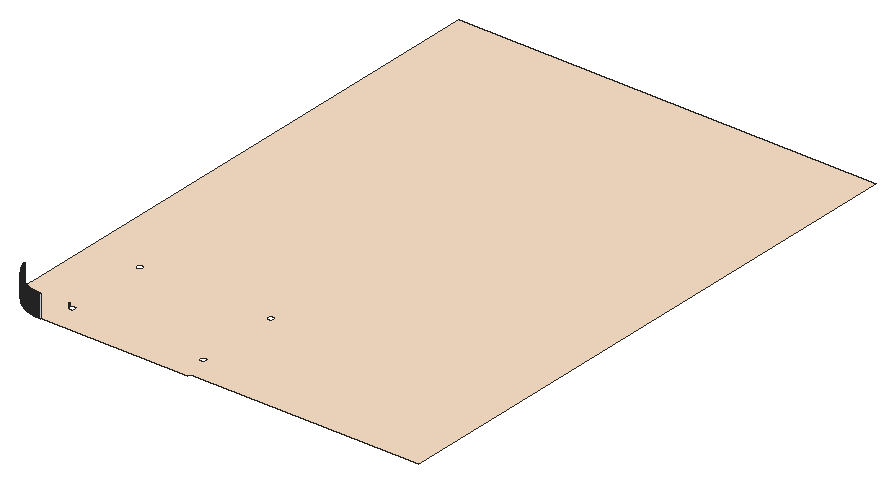
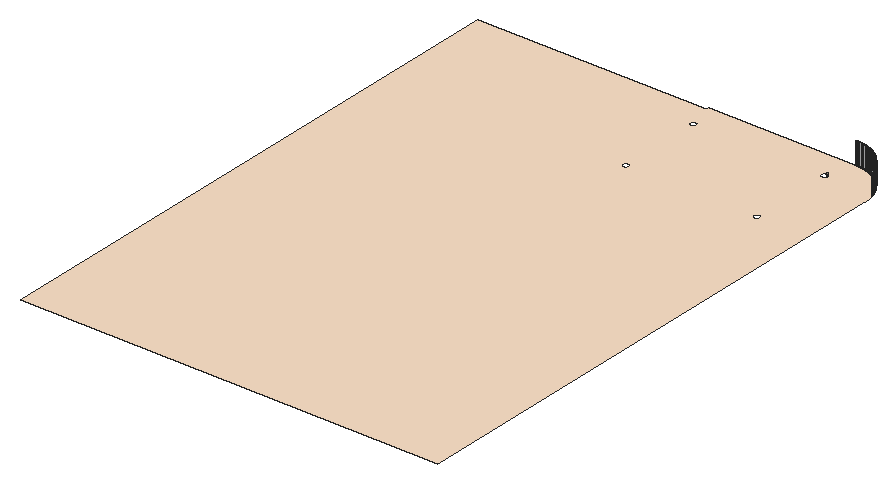
# SketchUp Ruby script. Lengths in inches.
U = 1.inch
M = Sketchup.active_model
def pt(a) = Geom::Point3d.new(a.map { |v| v * U })
def face(e, loops, mat)
  f = e.add_face(loops[0].map { |a| pt(a) })
  loops[1..].each { |l| e.add_face(l.map { |a| pt(a) }).erase! }
  f.material = f.back_material = mat if mat
  f
end
# faces: each face lists its corners as indices into pts; further lists are holes
def faces(e, pts, list, mat = nil) = list.each { |f| face(e, (f[0].is_a?(Array) ? f : [f]).map { |l| l.map { |i| pts[i] } }, mat) }
# xy, xz, yz: faces in a plane at the given z, y or x. An outline is a flat list of corners, or four numbers for a rectangle; further outlines are holes
def ring(l) = l.size == 4 ? [[l[0], l[1]], [l[2], l[1]], [l[2], l[3]], [l[0], l[3]]] : l.each_slice(2).to_a
def flat(e, list, mat, &to3) = list.each { |f| face(e, (f[0].is_a?(Array) ? f : [f]).map { |l| ring(l).map { |u, v| to3.(u, v) } }, mat) }
def xy(e, z, list, mat = nil) = flat(e, list, mat) { |x, y| [x, y, z] }
def xz(e, y, list, mat = nil) = flat(e, list, mat) { |x, z| [x, y, z] }
def yz(e, x, list, mat = nil) = flat(e, list, mat) { |y, z| [x, y, z] }
def lines(e, pts, list) = list.each { |a, b| e.add_line(pt(pts[a]), pt(pts[b])) }
# prism: a flat outline (further loops are holes) pulled along v
def prism(e, loops, v, mat = nil)
  f = face(e, loops, mat); d = Geom::Vector3d.new(v.map { |x| x * U })
  f.pushpull(f.normal.samedirection?(d) ? d.length : -d.length)
end
def box(e, o, s, mat = nil) = prism(e, [[o, [o[0] + s[0], o[1], o[2]], [o[0] + s[0], o[1] + s[1], o[2]], [o[0], o[1] + s[1], o[2]]]], [0, 0, s[2]], mat)
def at(x, y, z, deg = 0) = Geom::Transformation.translation(pt([x, y, z])) * Geom::Transformation.rotation(ORIGIN, Z_AXIS, deg.degrees)
def axes(o, x, y, z) = Geom::Transformation.new([*x, 0, *y, 0, *z, 0, *pt(o).to_a, 1])
def part(name) = M.definitions.add(name)
# library, detail: a bought-in or finely detailed component or shape, given as its bounding box
def library(name, o, s) = part(name).tap { |d| box(d.entities, o, s) }
def detail(e, o, s) = box(e.add_group.entities, o, s)
def put(e, d, t, mat = nil) = e.add_instance(d, t).tap { |i| i.material = mat if mat }
def group(e, t, mat = nil) = e.add_group.tap { |g| g.transformation = t; g.material = mat if mat }.entities
root = M.entities
M.materials.add("1122 AP 7994 PEACH ROSE").color = [254, 227, 201]
M.materials.add("[Quartz Light Grey]").color = [251, 251, 252]
xy(root,278.82,[[[44.6875,153,44.37,153.01,44.06,153.01,43.74,153.02,43.43,153.03,43.12,153.05,42.8,153.07,42.18,153.11,41.86,153.14,41.24,153.2,40.92,153.23,39.99,153.35,39.68,153.4,39.37,153.44,39.06,153.49,38.75,153.55,38.44,153.6,37.82,153.72,37.52,153.79,37.21,153.85,36.9,153.92,36.6,153.99,36.29,154.07,35.99,154.15,35.68,154.23,35.08,154.39,34.78,154.48,34.47,154.57,34.17,154.67,33.875,154.76,33.58,154.86,32.98,155.06,32.6875,155.17,32.39,155.28,31.81,155.5,31.51,155.62,30.93,155.86,30.65,155.99,30.36,156.11,30.07,156.24,29.79,156.37,29.5,156.51,29.22,156.64,28.9375,156.78,28.66,156.92,28.38,157.07,28.1,157.21,27.82,157.36,27.55,157.51,27.27,157.67,27,157.82,26.19,158.3,25.92,158.47,25.66,158.64,25.39,158.81,24.87,159.15,24.09,159.69,23.84,159.875,23.59,160.0625,23.33,160.25,23.08,160.4375,22.84,160.63,22.59,160.83,22.34,161.02,21.86,161.42,21.38,161.83,21.15,162.04,20.91,162.25,20.45,162.67,20.22,162.89,19.99,163.1,19.77,163.32,19.54,163.54,19.32,163.77,19.1,163.99,18.89,164.22,18.67,164.45,18.25,164.91,18.04,165.15,17.83,165.38,17.42,165.86,17.02,166.34,16.83,166.59,16.63,166.84,16.4375,167.08,16.25,167.33,16.0625,167.59,15.875,167.84,15.69,168.09,15.15,168.87,14.81,169.39,14.64,169.66,14.47,169.92,14.3,170.19,13.82,171,13.67,171.27,13.51,171.55,13.36,171.82,13.21,172.1,13.07,172.38,12.92,172.66,12.78,172.9375,12.64,173.22,12.51,173.5,12.37,173.79,12.24,174.07,12.11,174.36,11.99,174.65,11.86,174.93,11.62,175.51,11.5,175.81,11.28,176.39,11.17,176.6875,11.06,176.98,10.86,177.58,10.76,177.875,10.67,178.17,10.57,178.47,10.48,178.78,10.39,179.08,10.23,179.68,10.15,179.99,10.07,180.29,9.99,180.6,9.92,180.9,9.85,181.21,9.79,181.52,9.72,181.82,9.6,182.44,9.55,182.75,9.49,183.06,9.44,183.37,9.4,183.68,9.35,183.99,9.23,184.92,9.2,185.24,9.14,185.86,9.11,186.18,9.07,186.8,9.05,187.12,9.03,187.43,9.02,187.74,9.01,188.06,9.01,188.37,9,188.6875,9,645,366,645,366,156,171.19,156,171.19,153],[52.82,174,53.14,174,53.22,174.01,53.29,174.02,53.53,174.05,53.6,174.07,53.68,174.08,53.76,174.1,53.83,174.125,53.91,174.15,53.98,174.17,54.06,174.2,54.27,174.29,54.34,174.33,54.41,174.36,54.55,174.44,54.61,174.48,54.68,174.53,54.74,174.57,54.81,174.62,55.05,174.82,55.1,174.88,55.16,174.93,55.26,175.05,55.3125,175.11,55.36,175.17,55.41,175.24,55.45,175.3,55.5,175.37,55.54,175.43,55.62,175.57,55.65,175.64,55.6875,175.71,55.72,175.78,55.78,175.92,55.81,176,55.83,176.07,55.86,176.15,55.88,176.22,55.9,176.3,55.92,176.375,55.93,176.45,55.94,176.53,55.96,176.61,55.96,176.6875,55.97,176.76,55.98,176.84,55.98,177.16,55.97,177.24,55.96,177.3125,55.96,177.39,55.94,177.47,55.93,177.55,55.92,177.625,55.9,177.7,55.88,177.78,55.86,177.85,55.83,177.93,55.81,178,55.78,178.08,55.72,178.22,55.6875,178.29,55.65,178.36,55.62,178.43,55.54,178.57,55.5,178.63,55.45,178.7,55.41,178.76,55.36,178.83,55.3125,178.89,55.26,178.95,55.16,179.07,55.1,179.12,55.05,179.18,54.81,179.38,54.74,179.43,54.68,179.47,54.61,179.52,54.55,179.56,54.41,179.64,54.34,179.67,54.27,179.71,54.06,179.8,53.98,179.83,53.91,179.85,53.83,179.875,53.76,179.9,53.68,179.92,53.6,179.93,53.53,179.95,53.29,179.98,53.22,179.99,53.14,180,52.82,180,52.75,179.99,52.43,179.95,52.36,179.93,52.28,179.92,52.2,179.9,52.13,179.875,52.05,179.85,51.98,179.83,51.91,179.8,51.83,179.77,51.76,179.74,51.6875,179.71,51.62,179.67,51.55,179.64,51.41,179.56,51.35,179.52,51.28,179.47,51.22,179.43,51.15,179.38,50.97,179.23,50.86,179.12,50.8,179.07,50.6,178.83,50.55,178.76,50.51,178.7,50.46,178.63,50.42,178.57,50.34,178.43,50.31,178.36,50.27,178.29,50.18,178.08,50.15,178,50.13,177.93,50.1,177.85,50.08,177.78,50.0625,177.7,50.05,177.625,50.03,177.55,50.01,177.39,50,177.3125,49.99,177.24,49.99,177.16,49.98,177.08,49.98,176.92,49.99,176.84,49.99,176.76,50,176.6875,50.01,176.61,50.03,176.45,50.05,176.375,50.0625,176.3,50.08,176.22,50.1,176.15,50.13,176.07,50.15,176,50.18,175.92,50.27,175.71,50.31,175.64,50.34,175.57,50.42,175.43,50.46,175.37,50.51,175.3,50.55,175.24,50.6,175.17,50.8,174.93,50.86,174.88,50.97,174.77,51.15,174.62,51.22,174.57,51.28,174.53,51.35,174.48,51.41,174.44,51.55,174.36,51.62,174.33,51.6875,174.29,51.76,174.26,51.83,174.23,51.91,174.2,51.98,174.17,52.05,174.15,52.13,174.125,52.2,174.1,52.28,174.08,52.36,174.07,52.43,174.05,52.75,174.01],[164.84,246,165.16,246,165.24,246.01,165.3125,246.02,165.39,246.03,165.55,246.05,165.625,246.07,165.7,246.08,165.78,246.1,165.85,246.125,165.93,246.15,166,246.17,166.08,246.2,166.29,246.29,166.36,246.33,166.43,246.36,166.57,246.44,166.63,246.48,166.7,246.53,166.76,246.57,166.83,246.62,167.07,246.82,167.12,246.88,167.18,246.93,167.38,247.17,167.43,247.24,167.47,247.3,167.52,247.37,167.56,247.43,167.64,247.57,167.67,247.64,167.71,247.71,167.8,247.92,167.83,248,167.85,248.07,167.875,248.15,167.9,248.22,167.92,248.3,167.93,248.375,167.95,248.45,167.97,248.61,167.98,248.6875,167.99,248.76,168,248.84,168,249.16,167.99,249.24,167.98,249.3125,167.97,249.39,167.95,249.55,167.93,249.625,167.92,249.7,167.9,249.78,167.875,249.85,167.85,249.93,167.83,250,167.8,250.08,167.71,250.29,167.67,250.36,167.64,250.43,167.56,250.57,167.52,250.63,167.47,250.7,167.43,250.76,167.38,250.83,167.18,251.07,167.12,251.12,167.07,251.18,166.83,251.38,166.76,251.43,166.7,251.47,166.63,251.52,166.57,251.56,166.43,251.64,166.36,251.67,166.29,251.71,166.08,251.8,166,251.83,165.93,251.85,165.85,251.875,165.78,251.9,165.7,251.92,165.625,251.93,165.55,251.95,165.39,251.97,165.3125,251.98,165.24,251.99,165.16,252,164.84,252,164.76,251.99,164.6875,251.98,164.61,251.97,164.45,251.95,164.375,251.93,164.3,251.92,164.22,251.9,164.15,251.875,164.07,251.85,164,251.83,163.92,251.8,163.71,251.71,163.64,251.67,163.57,251.64,163.43,251.56,163.37,251.52,163.3,251.47,163.24,251.43,163.17,251.38,162.93,251.18,162.88,251.12,162.82,251.07,162.62,250.83,162.57,250.76,162.53,250.7,162.48,250.63,162.44,250.57,162.36,250.43,162.33,250.36,162.29,250.29,162.2,250.08,162.17,250,162.15,249.93,162.125,249.85,162.1,249.78,162.08,249.7,162.07,249.625,162.05,249.55,162.03,249.39,162.02,249.3125,162.01,249.24,162,249.16,162,248.84,162.01,248.76,162.02,248.6875,162.03,248.61,162.05,248.45,162.07,248.375,162.08,248.3,162.1,248.22,162.125,248.15,162.15,248.07,162.17,248,162.2,247.92,162.29,247.71,162.33,247.64,162.36,247.57,162.44,247.43,162.48,247.37,162.53,247.3,162.57,247.24,162.62,247.17,162.82,246.93,162.88,246.88,162.93,246.82,163.17,246.62,163.24,246.57,163.3,246.53,163.37,246.48,163.43,246.44,163.57,246.36,163.64,246.33,163.71,246.29,163.92,246.2,164,246.17,164.07,246.15,164.15,246.125,164.22,246.1,164.3,246.08,164.375,246.07,164.45,246.05,164.61,246.03,164.6875,246.02,164.76,246.01],[164.84,174,165.16,174,165.24,174.01,165.3125,174.02,165.39,174.03,165.55,174.05,165.625,174.07,165.7,174.08,165.78,174.1,165.85,174.125,165.93,174.15,166,174.17,166.08,174.2,166.29,174.29,166.36,174.33,166.43,174.36,166.57,174.44,166.63,174.48,166.7,174.53,166.76,174.57,166.83,174.62,167.07,174.82,167.12,174.88,167.18,174.93,167.38,175.17,167.43,175.24,167.47,175.3,167.52,175.37,167.56,175.43,167.64,175.57,167.67,175.64,167.71,175.71,167.8,175.92,167.83,176,167.85,176.07,167.875,176.15,167.9,176.22,167.92,176.3,167.93,176.375,167.95,176.45,167.97,176.61,167.98,176.6875,167.99,176.76,168,176.84,168,177.16,167.99,177.24,167.98,177.3125,167.97,177.39,167.95,177.55,167.93,177.625,167.92,177.7,167.9,177.78,167.875,177.85,167.85,177.93,167.83,178,167.8,178.08,167.71,178.29,167.67,178.36,167.64,178.43,167.56,178.57,167.52,178.63,167.47,178.7,167.43,178.76,167.38,178.83,167.18,179.07,167.12,179.12,167.07,179.18,166.83,179.38,166.76,179.43,166.7,179.47,166.63,179.52,166.57,179.56,166.43,179.64,166.36,179.67,166.29,179.71,166.08,179.8,166,179.83,165.93,179.85,165.85,179.875,165.78,179.9,165.7,179.92,165.625,179.93,165.55,179.95,165.39,179.97,165.3125,179.98,165.24,179.99,165.16,180,164.84,180,164.76,179.99,164.6875,179.98,164.61,179.97,164.45,179.95,164.375,179.93,164.3,179.92,164.22,179.9,164.15,179.875,164.07,179.85,164,179.83,163.92,179.8,163.71,179.71,163.64,179.67,163.57,179.64,163.43,179.56,163.37,179.52,163.3,179.47,163.24,179.43,163.17,179.38,162.93,179.18,162.88,179.12,162.82,179.07,162.62,178.83,162.57,178.76,162.53,178.7,162.48,178.63,162.44,178.57,162.36,178.43,162.33,178.36,162.29,178.29,162.2,178.08,162.17,178,162.15,177.93,162.125,177.85,162.1,177.78,162.08,177.7,162.07,177.625,162.05,177.55,162.03,177.39,162.02,177.3125,162.01,177.24,162,177.16,162,176.84,162.01,176.76,162.02,176.6875,162.03,176.61,162.05,176.45,162.07,176.375,162.08,176.3,162.1,176.22,162.125,176.15,162.15,176.07,162.17,176,162.2,175.92,162.29,175.71,162.33,175.64,162.36,175.57,162.44,175.43,162.48,175.37,162.53,175.3,162.57,175.24,162.62,175.17,162.82,174.93,162.88,174.88,162.93,174.82,163.17,174.62,163.24,174.57,163.3,174.53,163.37,174.48,163.43,174.44,163.57,174.36,163.64,174.33,163.71,174.29,163.92,174.2,164,174.17,164.07,174.15,164.15,174.125,164.22,174.1,164.3,174.08,164.375,174.07,164.45,174.05,164.61,174.03,164.6875,174.02,164.76,174.01],[52.82,246,53.14,246,53.22,246.01,53.29,246.02,53.53,246.05,53.6,246.07,53.68,246.08,53.76,246.1,53.83,246.125,53.91,246.15,53.98,246.17,54.06,246.2,54.27,246.29,54.34,246.33,54.41,246.36,54.55,246.44,54.61,246.48,54.68,246.53,54.74,246.57,54.81,246.62,55.05,246.82,55.1,246.88,55.16,246.93,55.26,247.05,55.3125,247.11,55.36,247.17,55.41,247.24,55.45,247.3,55.5,247.37,55.54,247.43,55.62,247.57,55.65,247.64,55.6875,247.71,55.72,247.78,55.78,247.92,55.81,248,55.83,248.07,55.86,248.15,55.88,248.22,55.9,248.3,55.92,248.375,55.93,248.45,55.94,248.53,55.96,248.61,55.96,248.6875,55.97,248.76,55.98,248.84,55.98,249.16,55.97,249.24,55.96,249.3125,55.96,249.39,55.94,249.47,55.93,249.55,55.92,249.625,55.9,249.7,55.88,249.78,55.86,249.85,55.83,249.93,55.81,250,55.78,250.08,55.72,250.22,55.6875,250.29,55.65,250.36,55.62,250.43,55.54,250.57,55.5,250.63,55.45,250.7,55.41,250.76,55.36,250.83,55.3125,250.89,55.26,250.95,55.16,251.07,55.1,251.12,55.05,251.18,54.81,251.38,54.74,251.43,54.68,251.47,54.61,251.52,54.55,251.56,54.41,251.64,54.34,251.67,54.27,251.71,54.06,251.8,53.98,251.83,53.91,251.85,53.83,251.875,53.76,251.9,53.68,251.92,53.6,251.93,53.53,251.95,53.29,251.98,53.22,251.99,53.14,252,52.82,252,52.75,251.99,52.43,251.95,52.36,251.93,52.28,251.92,52.2,251.9,52.13,251.875,52.05,251.85,51.98,251.83,51.91,251.8,51.83,251.77,51.76,251.74,51.6875,251.71,51.62,251.67,51.55,251.64,51.41,251.56,51.35,251.52,51.28,251.47,51.22,251.43,51.15,251.38,50.97,251.23,50.86,251.12,50.8,251.07,50.6,250.83,50.55,250.76,50.51,250.7,50.46,250.63,50.42,250.57,50.34,250.43,50.31,250.36,50.27,250.29,50.18,250.08,50.15,250,50.13,249.93,50.1,249.85,50.08,249.78,50.0625,249.7,50.05,249.625,50.03,249.55,50.01,249.39,50,249.3125,49.99,249.24,49.99,249.16,49.98,249.08,49.98,248.92,49.99,248.84,49.99,248.76,50,248.6875,50.01,248.61,50.03,248.45,50.05,248.375,50.0625,248.3,50.08,248.22,50.1,248.15,50.13,248.07,50.15,248,50.18,247.92,50.27,247.71,50.31,247.64,50.34,247.57,50.42,247.43,50.46,247.37,50.51,247.3,50.55,247.24,50.6,247.17,50.8,246.93,50.86,246.88,50.97,246.77,51.15,246.62,51.22,246.57,51.28,246.53,51.35,246.48,51.41,246.44,51.55,246.36,51.62,246.33,51.6875,246.29,51.76,246.26,51.83,246.23,51.91,246.2,51.98,246.17,52.05,246.15,52.13,246.125,52.2,246.1,52.28,246.08,52.36,246.07,52.43,246.05,52.75,246.01]]],"1122 AP 7994 PEACH ROSE")
xz(root,153,[[44.6875,278.82,45,297.82]],"[Quartz Light Grey]")
xz(root,153.01,[[44.06,278.82,44.37,297.82]],"[Quartz Light Grey]")
yz(root,49.98,[[176.92,278.82,177,281.82],[177,278.82,177.08,281.82]],"1122 AP 7994 PEACH ROSE")
yz(root,49.99,[[176.76,278.82,176.84,281.82],[177.16,278.82,177.24,281.82]],"1122 AP 7994 PEACH ROSE")
p = [[42.8,153.07,278.82],[43.12,153.05,278.82],[43.12,153.05,297.82],[42.8,153.07,297.82],[43.43,153.03,278.82],[43.43,153.03,297.82],
  [43.74,153.02,278.82],[43.74,153.02,297.82],[44.06,153.01,278.82],[44.06,153.01,297.82],[44.37,153.01,278.82],[44.6875,153,278.82],
  [44.6875,153,297.82],[44.37,153.01,297.82],[41.55,153.17,278.82],[41.86,153.14,278.82],[41.86,153.14,297.82],[41.55,153.17,297.82],
  [42.18,153.11,278.82],[42.18,153.11,297.82],[42.49,153.09,278.82],[42.49,153.09,297.82],[40.61,153.27,278.82],[40.92,153.23,278.82],
  [40.92,153.23,297.82],[40.61,153.27,297.82],[41.24,153.2,278.82],[41.24,153.2,297.82],[39.99,153.35,278.82],[40.3,153.31,278.82],
  [40.3,153.31,297.82],[39.99,153.35,297.82],[39.06,153.49,278.82],[39.37,153.44,278.82],[39.37,153.44,297.82],[39.06,153.49,297.82],
  [39.68,153.4,278.82],[39.68,153.4,297.82],[38.44,153.6,278.82],[38.75,153.55,278.82],[38.75,153.55,297.82],[38.44,153.6,297.82],
  [38.13,153.66,278.82],[38.13,153.66,297.82],[37.52,153.79,278.82],[37.82,153.72,278.82],[37.82,153.72,297.82],[37.52,153.79,297.82],
  [37.21,153.85,278.82],[37.21,153.85,297.82],[36.6,153.99,278.82],[36.9,153.92,278.82],[36.9,153.92,297.82],[36.6,153.99,297.82],
  [36.29,154.07,278.82],[36.29,154.07,297.82],[35.68,154.23,278.82],[35.99,154.15,278.82],[35.99,154.15,297.82],[35.68,154.23,297.82],
  [35.38,154.31,278.82],[35.38,154.31,297.82],[35.08,154.39,278.82],[35.08,154.39,297.82],[34.78,154.48,278.82],[34.78,154.48,297.82],
  [34.47,154.57,278.82],[34.47,154.57,297.82],[34.17,154.67,278.82],[34.17,154.67,297.82],[33.875,154.76,278.82],[33.875,154.76,297.82],
  [33.58,154.86,278.82],[33.58,154.86,297.82],[33.28,154.96,278.82],[33.28,154.96,297.82],[32.98,155.06,278.82],[32.98,155.06,297.82],
  [32.6875,155.17,278.82],[32.6875,155.17,297.82],[32.39,155.28,278.82],[32.39,155.28,297.82],[32.1,155.39,278.82],[32.1,155.39,297.82],
  [31.81,155.5,278.82],[31.81,155.5,297.82],[31.51,155.62,278.82],[31.51,155.62,297.82],[31.22,155.74,278.82],[31.22,155.74,297.82],
  [30.93,155.86,278.82],[30.93,155.86,297.82],[30.65,155.99,278.82],[30.65,155.99,297.82],[30.36,156.11,278.82],[30.36,156.11,297.82],
  [30.07,156.24,278.82],[30.07,156.24,297.82],[29.79,156.37,278.82],[29.79,156.37,297.82],[29.5,156.51,278.82],[29.5,156.51,297.82],
  [29.22,156.64,278.82],[29.22,156.64,297.82],[28.9375,156.78,278.82],[28.9375,156.78,297.82],[28.66,156.92,278.82],[28.66,156.92,297.82],
  [28.38,157.07,278.82],[28.38,157.07,297.82],[28.1,157.21,278.82],[28.1,157.21,297.82],[27.82,157.36,278.82],[27.82,157.36,297.82],
  [27.55,157.51,278.82],[27.55,157.51,297.82],[27.27,157.67,278.82],[27.27,157.67,297.82],[27,157.82,278.82],[27,157.82,297.82],
  [26.73,157.98,278.82],[26.73,157.98,297.82],[26.46,158.14,278.82],[26.46,158.14,297.82],[26.19,158.3,278.82],[26.19,158.3,297.82],
  [25.92,158.47,278.82],[25.92,158.47,297.82],[25.66,158.64,278.82],[25.66,158.64,297.82],[25.39,158.81,278.82],[25.39,158.81,297.82],
  [25.13,158.98,278.82],[25.13,158.98,297.82],[24.87,159.15,278.82],[24.87,159.15,297.82],[24.61,159.33,278.82],[24.61,159.33,297.82],
  [24.35,159.51,278.82],[24.35,159.51,297.82],[24.09,159.69,278.82],[24.09,159.69,297.82],[23.84,159.875,278.82],[23.84,159.875,297.82],
  [23.59,160.0625,278.82],[23.59,160.0625,297.82],[23.33,160.25,278.82],[23.33,160.25,297.82],[23.08,160.4375,278.82],[23.08,160.4375,297.82],
  [22.84,160.63,278.82],[22.84,160.63,297.82],[22.59,160.83,278.82],[22.59,160.83,297.82],[22.34,161.02,278.82],[22.34,161.02,297.82],
  [22.1,161.22,278.82],[22.1,161.22,297.82],[21.86,161.42,278.82],[21.86,161.42,297.82],[21.62,161.625,278.82],[21.62,161.625,297.82],
  [21.38,161.83,278.82],[21.38,161.83,297.82],[21.15,162.04,278.82],[21.15,162.04,297.82],[20.91,162.25,278.82],[20.91,162.25,297.82],
  [20.68,162.46,278.82],[20.68,162.46,297.82],[20.45,162.67,278.82],[20.45,162.67,297.82],[20.22,162.89,278.82],[20.22,162.89,297.82],
  [19.99,163.1,278.82],[19.99,163.1,297.82],[19.77,163.32,278.82],[19.77,163.32,297.82],[19.54,163.54,278.82],[19.54,163.54,297.82],
  [19.32,163.77,278.82],[19.32,163.77,297.82],[19.1,163.99,278.82],[19.1,163.99,297.82],[18.89,164.22,278.82],[18.89,164.22,297.82],
  [18.67,164.45,278.82],[18.67,164.45,297.82],[18.46,164.68,278.82],[18.46,164.68,297.82],[18.25,164.91,278.82],[18.25,164.91,297.82],
  [18.04,165.15,278.82],[18.04,165.15,297.82],[17.83,165.38,278.82],[17.83,165.38,297.82],[17.625,165.62,278.82],[17.625,165.62,297.82],
  [17.42,165.86,278.82],[17.42,165.86,297.82],[17.22,166.1,278.82],[17.22,166.1,297.82],[17.02,166.34,278.82],[17.02,166.34,297.82],
  [16.83,166.59,278.82],[16.83,166.59,297.82],[16.63,166.84,278.82],[16.63,166.84,297.82],[16.4375,167.08,278.82],[16.4375,167.08,297.82],
  [16.25,167.33,278.82],[16.25,167.33,297.82],[16.0625,167.59,278.82],[16.0625,167.59,297.82],[15.875,167.84,278.82],[15.875,167.84,297.82],
  [15.69,168.09,278.82],[15.69,168.09,297.82],[15.51,168.35,278.82],[15.51,168.35,297.82],[15.33,168.61,278.82],[15.33,168.61,297.82],
  [15.15,168.87,278.82],[15.15,168.87,297.82],[14.98,169.13,278.82],[14.98,169.13,297.82],[14.81,169.39,278.82],[14.81,169.39,297.82],
  [14.64,169.66,278.82],[14.64,169.66,297.82],[14.47,169.92,278.82],[14.47,169.92,297.82],[14.3,170.19,278.82],[14.3,170.19,297.82],
  [14.14,170.46,278.82],[14.14,170.46,297.82],[13.98,170.73,278.82],[13.98,170.73,297.82],[13.82,171,278.82],[13.82,171,297.82],
  [13.67,171.27,278.82],[13.67,171.27,297.82],[13.51,171.55,278.82],[13.51,171.55,297.82],[13.36,171.82,278.82],[13.36,171.82,297.82],
  [13.21,172.1,278.82],[13.21,172.1,297.82],[13.07,172.38,278.82],[13.07,172.38,297.82],[12.92,172.66,278.82],[12.92,172.66,297.82],
  [12.78,172.9375,278.82],[12.78,172.9375,297.82],[12.64,173.22,278.82],[12.64,173.22,297.82],[12.51,173.5,278.82],[12.51,173.5,297.82],
  [12.37,173.79,278.82],[12.37,173.79,297.82],[12.24,174.07,278.82],[12.24,174.07,297.82],[12.11,174.36,278.82],[12.11,174.36,297.82],
  [11.99,174.65,278.82],[11.99,174.65,297.82],[11.86,174.93,278.82],[11.86,174.93,297.82],[11.74,175.22,278.82],[11.74,175.22,297.82],
  [11.62,175.51,278.82],[11.62,175.51,297.82],[11.5,175.81,278.82],[11.5,175.81,297.82],[11.39,176.1,278.82],[11.39,176.1,297.82],
  [11.28,176.39,278.82],[11.28,176.39,297.82],[11.17,176.6875,278.82],[11.17,176.6875,297.82],[50.02,176.53,278.82],[50.01,176.61,278.82],
  [50.01,176.61,281.82],[50.02,176.53,281.82],[50.03,176.45,278.82],[50.03,176.45,281.82],[50,176.6875,278.82],[50,176.6875,281.82],
  [11.06,176.98,278.82],[11.06,176.98,297.82],[49.99,176.76,278.82],[49.99,176.76,281.82],[49.99,176.84,278.82],[49.98,176.92,278.82],
  [49.98,176.92,281.82],[49.99,176.84,281.82],[10.96,177.28,278.82],[10.96,177.28,297.82],[49.98,177.08,278.82],[49.99,177.16,278.82],
  [49.99,177.16,281.82],[49.98,177.08,281.82],[49.99,177.24,278.82],[50,177.3125,278.82],[50,177.3125,281.82],[49.99,177.24,281.82],
  [10.86,177.58,278.82],[10.86,177.58,297.82],[50.01,177.39,278.82],[50.01,177.39,281.82],[50.02,177.47,278.82],[50.02,177.47,281.82],
  [10.76,177.875,278.82],[10.76,177.875,297.82],[10.67,178.17,278.82],[10.67,178.17,297.82],[10.57,178.47,278.82],[10.57,178.47,297.82],
  [10.48,178.78,278.82],[10.48,178.78,297.82],[10.39,179.08,278.82],[10.39,179.08,297.82]]
faces(root,p,[[0,1,2,3],[1,4,5,2],[4,6,7,5],[6,8,9,7],[10,11,12,13],[14,15,16,17],[15,18,19,16],[18,20,21,19],
  [20,0,3,21],[22,23,24,25],[23,26,27,24],[26,14,17,27],[28,29,30,31],[29,22,25,30],[32,33,34,35],[33,36,37,34],
  [36,28,31,37],[38,39,40,41],[39,32,35,40],[42,38,41,43],[44,45,46,47],[45,42,43,46],[48,44,47,49],[50,51,52,53],
  [51,48,49,52],[54,50,53,55],[56,57,58,59],[57,54,55,58],[60,56,59,61],[62,60,61,63],[64,62,63,65],[66,64,65,67],
  [68,66,67,69],[70,68,69,71],[72,70,71,73],[74,72,73,75],[76,74,75,77],[78,76,77,79],[80,78,79,81],[82,80,81,83],
  [84,82,83,85],[86,84,85,87],[88,86,87,89],[90,88,89,91],[92,90,91,93],[94,92,93,95],[96,94,95,97],[98,96,97,99],
  [100,98,99,101],[102,100,101,103],[104,102,103,105],[106,104,105,107],[108,106,107,109],[110,108,109,111],[112,110,111,113],[114,112,113,115],
  [116,114,115,117],[118,116,117,119],[120,118,119,121],[122,120,121,123],[124,122,123,125],[126,124,125,127],[128,126,127,129],[130,128,129,131],
  [132,130,131,133],[134,132,133,135],[136,134,135,137],[138,136,137,139],[140,138,139,141],[142,140,141,143],[144,142,143,145],[146,144,145,147],
  [148,146,147,149],[150,148,149,151],[152,150,151,153],[154,152,153,155],[156,154,155,157],[158,156,157,159],[160,158,159,161],[162,160,161,163],
  [164,162,163,165],[166,164,165,167],[168,166,167,169],[170,168,169,171],[172,170,171,173],[174,172,173,175],[176,174,175,177],[178,176,177,179],
  [180,178,179,181],[182,180,181,183],[184,182,183,185],[186,184,185,187],[188,186,187,189],[190,188,189,191],[192,190,191,193],[194,192,193,195],
  [196,194,195,197],[198,196,197,199],[200,198,199,201],[202,200,201,203],[204,202,203,205],[206,204,205,207],[208,206,207,209],[210,208,209,211],
  [212,210,211,213],[214,212,213,215],[216,214,215,217],[218,216,217,219],[220,218,219,221],[222,220,221,223],[224,222,223,225],[226,224,225,227],
  [228,226,227,229],[230,228,229,231],[232,230,231,233],[234,232,233,235],[236,234,235,237],[238,236,237,239],[240,238,239,241],[242,240,241,243],
  [244,242,243,245],[246,244,245,247],[248,246,247,249],[250,248,249,251],[252,250,251,253],[254,252,253,255],[256,254,255,257],[258,256,257,259],
  [260,258,259,261],[262,260,261,263],[264,262,263,265],[266,264,265,267],[268,266,267,269],[270,268,269,271],[272,270,271,273],[274,272,273,275],
  [276,274,275,277],[278,276,277,279],[288,278,279,289],[296,288,289,297],[306,296,297,307],[312,306,307,313],[314,312,313,315],[316,314,315,317],
  [318,316,317,319],[320,318,319,321]],"[Quartz Light Grey]")
faces(root,p,[[280,281,282,283],[284,280,283,285],[281,286,287,282],[286,290,291,287],[292,293,294,295],[298,299,300,301],[302,303,304,305],[303,308,309,304],
  [308,310,311,309]],"1122 AP 7994 PEACH ROSE")
